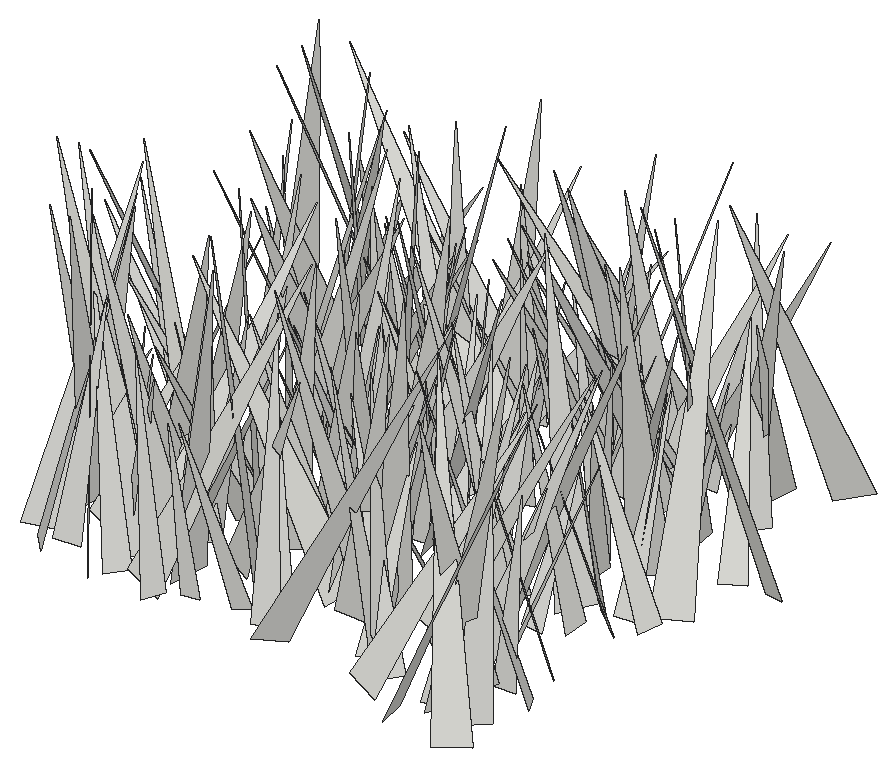
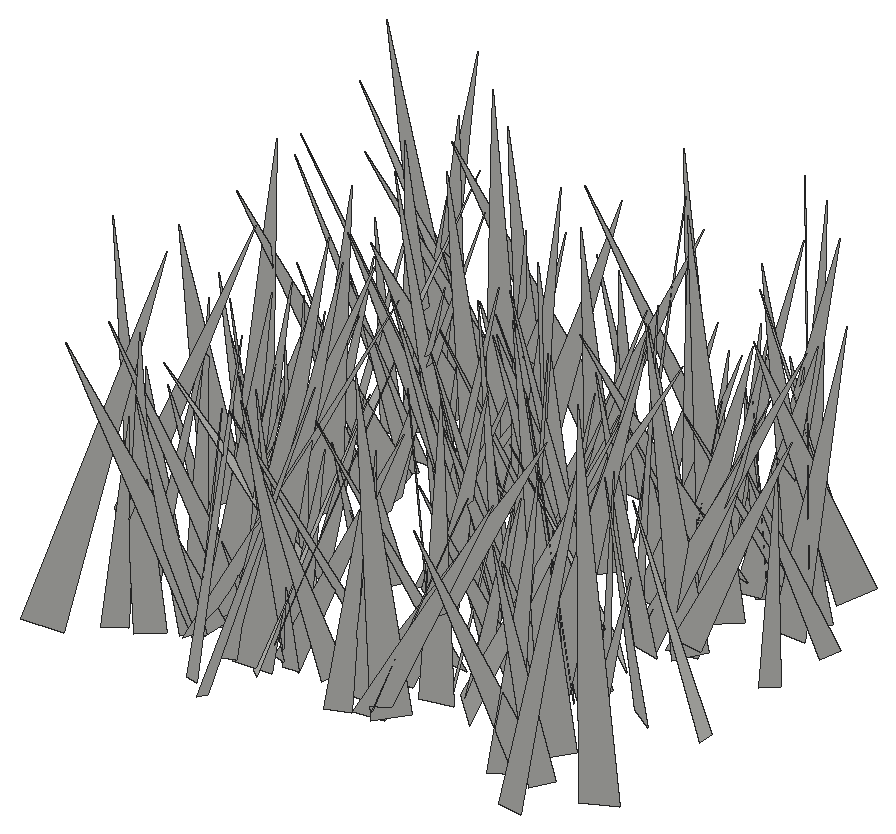
# SketchUp Ruby script. Lengths in inches.
U = 1.inch
M = Sketchup.active_model
def pt(a) = Geom::Point3d.new(a.map { |v| v * U })
def face(e, loops, mat)
  f = e.add_face(loops[0].map { |a| pt(a) })
  loops[1..].each { |l| e.add_face(l.map { |a| pt(a) }).erase! }
  f.material = f.back_material = mat if mat
  f
end
# faces: each face lists its corners as indices into pts; further lists are holes
def faces(e, pts, list, mat = nil) = list.each { |f| face(e, (f[0].is_a?(Array) ? f : [f]).map { |l| l.map { |i| pts[i] } }, mat) }
# xy, xz, yz: faces in a plane at the given z, y or x. An outline is a flat list of corners, or four numbers for a rectangle; further outlines are holes
def ring(l) = l.size == 4 ? [[l[0], l[1]], [l[2], l[1]], [l[2], l[3]], [l[0], l[3]]] : l.each_slice(2).to_a
def flat(e, list, mat, &to3) = list.each { |f| face(e, (f[0].is_a?(Array) ? f : [f]).map { |l| ring(l).map { |u, v| to3.(u, v) } }, mat) }
def xy(e, z, list, mat = nil) = flat(e, list, mat) { |x, y| [x, y, z] }
def xz(e, y, list, mat = nil) = flat(e, list, mat) { |x, z| [x, y, z] }
def yz(e, x, list, mat = nil) = flat(e, list, mat) { |y, z| [x, y, z] }
def lines(e, pts, list) = list.each { |a, b| e.add_line(pt(pts[a]), pt(pts[b])) }
# prism: a flat outline (further loops are holes) pulled along v
def prism(e, loops, v, mat = nil)
  f = face(e, loops, mat); d = Geom::Vector3d.new(v.map { |x| x * U })
  f.pushpull(f.normal.samedirection?(d) ? d.length : -d.length)
end
def box(e, o, s, mat = nil) = prism(e, [[o, [o[0] + s[0], o[1], o[2]], [o[0] + s[0], o[1] + s[1], o[2]], [o[0], o[1] + s[1], o[2]]]], [0, 0, s[2]], mat)
def at(x, y, z, deg = 0) = Geom::Transformation.translation(pt([x, y, z])) * Geom::Transformation.rotation(ORIGIN, Z_AXIS, deg.degrees)
def axes(o, x, y, z) = Geom::Transformation.new([*x, 0, *y, 0, *z, 0, *pt(o).to_a, 1])
def part(name) = M.definitions.add(name)
# library, detail: a bought-in or finely detailed component or shape, given as its bounding box
def library(name, o, s) = part(name).tap { |d| box(d.entities, o, s) }
def detail(e, o, s) = box(e.add_group.entities, o, s)
def put(e, d, t, mat = nil) = e.add_instance(d, t).tap { |i| i.material = mat if mat }
def group(e, t, mat = nil) = e.add_group.tap { |g| g.transformation = t; g.material = mat if mat }.entities
root = M.entities
c1 = part("fur_instance\#9")
p = [[0.8125,0,1.79],[0.67,-0.02,1.48],[0,-0.11,0],[0,0.11,0]]
faces(c1.entities,p,[[0,1,2,3]])
put(root,c1,axes([134.09,378.43,-27.1],[5.76412,-4.56343,1.38579],[-4.26746,-5.90574,-1.69745],[-2.12934,-0.51736,7.15322]))
put(root,c1,axes([135.99,374.47,-27.1],[-2.86004,7.00076,0.77945],[7.00763,2.7424,1.08181],[-0.71502,-1.12544,7.48466]))
put(root,c1,axes([132.64,375.04,-27.1],[7.12948,2.21776,0.41944],[2.17259,-7.11974,0.71624],[-0.61174,0.56098,7.43203]))
put(root,c1,axes([133.92,376.66,-27.1],[7.67247,-2.21843,2.0813],[-2.41925,-7.8734,0.52613],[-1.84403,1.09916,7.96941]))
put(root,c1,axes([116.74,376.78,-27.1],[-5.8561,-4.67693,3.47291],[-5.12361,6.47844,0.0849],[2.77191,2.09401,7.49403]))
put(root,c1,axes([120.1,376.48,-27.1],[-4.33048,1.8912,1.2808],[1.94847,4.49129,-0.04381],[1.19187,-0.47097,4.72523]))
put(root,c1,axes([123.3,377.78,-27.1],[0.25989,-4.12749,1.06746],[-4.12688,-0.51192,-0.97467],[-1.06982,0.97209,4.01917]))
put(root,c1,axes([121.22,377.3,-27.1],[0.17752,-3.57602,1.3313],[-3.7929,-0.31113,-0.32997],[-0.41733,1.30655,3.56518]))
put(root,c1,axes([120.11,378.6,-27.1],[7.47084,-2.00529,1.5784],[-1.88161,-7.62701,-0.78379],[-1.72397,-0.36551,7.69548]))
put(root,c1,axes([130.46,376,-27.1],[1.42855,6.69806,0.59183],[6.31436,-1.12829,-2.47201],[2.31152,-1.05735,6.38701]))
put(root,c1,axes([125.57,376.6,-27.1],[7.23014,-2.66142,0.8801],[-2.79977,-6.73645,2.62947],[0.1379,2.76941,7.24182]))
put(root,c1,axes([130.05,377.68,-27.1],[-5.84783,-0.54956,0.92386],[-0.66437,5.86496,-0.71656],[0.84507,0.80798,5.82972]))
put(root,c1,axes([135.58,376.33,-27.1],[-6.65914,2.85732,1.17721],[2.6023,6.69305,-1.52492],[1.66678,0.96593,7.084]))
put(root,c1,axes([115.02,377.66,-27.1],[-0.99114,4.85366,1.48422],[5.00835,1.18049,-0.51592],[0.82303,-1.33855,4.92689]))
put(root,c1,axes([119.22,376.96,-27.1],[1.74287,7.71217,1.36191],[7.45298,-1.20484,-2.71503],[2.4053,-1.85492,7.42588]))
put(root,c1,axes([119.18,379.17,-27.1],[-7.26017,0.65472,1.63239],[0.85,7.37598,0.82207],[1.53976,-0.9847,7.24313]))
put(root,c1,axes([113.81,381.06,-27.1],[7.57168,-2.77915,1.4038],[-2.39268,-7.55557,-2.05259],[-1.99233,-1.48808,7.80006]))
put(root,c1,axes([117.86,377.12,-27.1],[-5.44212,1.96061,0.21811],[1.90755,5.39324,-0.88463],[0.50284,0.7598,5.71648]))
put(root,c1,axes([130.01,377.82,-27.1],[-5.54219,0.95074,1.40051],[0.80502,5.69802,-0.68242],[1.48905,0.4581,5.58158]))
put(root,c1,axes([124.8125,377.26,-27.1],[-0.46142,6.00885,1.03301],[6.04976,0.32253,0.82618],[-0.75742,-1.08443,5.96964]))
put(root,c1,axes([136.26,378.83,-27.1],[-5.87124,-3.56524,0.53214],[-3.58838,5.68376,-1.51131],[-0.34307,1.5651,6.70063]))
put(root,c1,axes([130.94,377.24,-27.1],[-1.18961,5.30841,0.21099],[4.92708,1.02155,2.07828],[-1.98686,-0.64508,5.02744]))
put(root,c1,axes([127,379.875,-27.1],[2.07554,-6.96607,1.71735],[-7.11885,-1.77704,1.39545],[0.89291,2.02467,7.13349]))
put(root,c1,axes([122.99,379.21,-27.1],[-6.35073,-3.49942,2.22612],[-3.7296,6.59945,-0.26567],[1.81428,1.31702,7.24617]))
put(root,c1,axes([134.78,379.1,-27.1],[-0.53957,3.97433,2.02364],[4.38519,0.84425,-0.48882],[0.81275,-1.91664,3.98089]))
put(root,c1,axes([114.22,377.01,-27.1],[5.15399,5.0376,1.12923],[4.93282,-5.27609,1.02292],[-1.5231,-0.04087,7.13405]))
put(root,c1,axes([124.59,378.55,-27.1],[-2.6188,2.85202,1.01974],[2.95253,2.70449,0.01846],[0.67563,-0.76402,3.87193]))
put(root,c1,axes([129.3,377.81,-27.1],[-2.23012,3.65012,0.738],[3.54975,2.34365,-0.86487],[1.12574,-0.15918,4.18913]))
put(root,c1,axes([116.7,379.11,-27.1],[2.33806,3.32528,1.40975],[3.5899,-2.32407,-0.47188],[-0.3968,-1.43269,4.03749]))
put(root,c1,axes([121.08,380.21,-27.1],[-0.06945,-5.66946,1.63507],[-5.27402,0.7929,2.5253],[2.64594,1.43164,5.07647]))
put(root,c1,axes([116.05,380.35,-27.1],[-0.58442,-4.16845,1.10453],[-3.96593,0.95723,1.51414],[1.69333,0.80327,3.92746]))
put(root,c1,axes([127.69,380.28,-27.1],[-1.28539,6.13898,3.44989],[6.89976,0.39684,1.86462],[-1.40785,-3.66012,5.98853]))
put(root,c1,axes([127.63,381.2,-27.1],[3.37968,-7.43588,1.46776],[-7.57694,-3.27406,0.85991],[0.19143,1.6903,8.12251]))
put(root,c1,axes([125.64,380.97,-27.1],[-6.93796,2.79801,1.11968],[3.01121,6.55067,2.28891],[0.12298,-2.54512,7.12215]))
put(root,c1,axes([116.3,380.35,-27.1],[-4.3642,6.37446,3.0679],[7.06974,4.05938,1.62241],[0.25406,-3.46117,7.553]))
put(root,c1,axes([135.3,381.24,-27.1],[-3.21192,-3.98216,0.77509],[-3.98629,3.28152,0.34045],[0.75355,0.38579,5.10471]))
put(root,c1,axes([133.55,376.53,-27.1],[-6.0414,2.82747,0.77084],[2.14541,5.47009,-3.25002],[1.99649,2.67784,5.82499]))
put(root,c1,axes([115.99,380.21,-27.1],[3.13173,2.6382,1.54856],[2.8558,-3.31576,-0.12654],[-1.0966,-1.10068,4.0929]))
put(root,c1,axes([113.33,380.84,-27.1],[4.2743,-5.66959,1.70794],[-5.91958,-4.14155,1.06631],[-0.14077,2.00854,7.01974]))
put(root,c1,axes([117.75,382.05,-27.1],[3.73697,-5.4189,0.58942],[-5.45085,-3.71358,0.41766],[0.01126,0.72231,6.56925]))
put(root,c1,axes([116.83,382.71,-27.1],[4.42124,-3.27,0.9733],[-2.9097,-4.44582,-1.71927],[-1.78153,-0.85401,5.22344]))
put(root,c1,axes([117.72,378.53,-27.1],[-0.98442,7.82804,0.7856],[7.24103,0.59195,3.17514],[-3.07617,-1.11168,7.22258]))
put(root,c1,axes([130.6,380.02,-27.1],[4.59981,5.90875,0.46757],[5.722,-4.27232,-2.30133],[1.54616,-1.76752,7.12569]))
put(root,c1,axes([113.44,378.05,-27.1],[-5.30404,4.85737,1.41696],[4.30663,5.41145,-2.42976],[2.65607,0.92563,6.76928]))
put(root,c1,axes([113.57,381.97,-27.1],[0.65749,-6.30029,1.7132],[-6.47052,-0.85883,-0.67511],[-0.87239,1.62165,6.29842]))
put(root,c1,axes([124.79,380.67,-27.1],[2.82445,3.52777,0.66946],[3.53756,-2.58781,-1.2883],[0.61561,-1.31488,4.33162]))
put(root,c1,axes([116.1,382.74,-27.1],[3.30529,-7.09092,0.75642],[-7.06387,-3.14139,1.41833],[0.97724,1.27626,7.69379]))
put(root,c1,axes([119.27,383.22,-27.1],[0.9036,-5.03288,0.01557],[-4.93923,-0.88981,-0.97923],[-0.96652,-0.158,5.01871]))
put(root,c1,axes([124.92,381.69,-27.1],[-5.6933,-0.47947,0.5538],[-0.44449,5.71072,0.37467],[0.58224,-0.32872,5.70116]))
put(root,c1,axes([118.86,381.36,-27.1],[4.80209,-1.99507,1.20954],[-2.10711,-4.89697,0.2883],[-1.00169,0.73669,5.19204]))
put(root,c1,axes([132.38,381.06,-27.1],[0.51441,-3.71167,1.78135],[-3.92489,0.09986,1.3415],[1.24297,1.85145,3.49879]))
put(root,c1,axes([132.69,380.19,-27.1],[2.40606,6.39383,1.08481],[6.38564,-2.13376,-1.58675],[1.13207,-1.55339,6.64473]))
put(root,c1,axes([114.79,379.82,-27.1],[1.15422,4.7345,0.08294],[4.6056,-1.10261,-1.15208],[1.10037,-0.35121,4.73502]))
put(root,c1,axes([118.68,380.27,-27.1],[4.79219,0.94532,0.41054],[0.81575,-4.67249,1.23678],[-0.62985,1.14081,4.72537]))
put(root,c1,axes([128.04,380.29,-27.1],[5.65388,1.0827,1.74004],[0.6959,-5.81697,1.3583],[-1.92762,1.07564,5.59407]))
put(root,c1,axes([121.86,382.43,-27.1],[5.17414,-4.36417,1.70527],[-4.54977,-5.28673,0.27499],[-1.1196,1.31532,6.76329]))
put(root,c1,axes([127.16,380.84,-27.1],[-1.66344,3.87519,0.54462],[3.91265,1.65754,0.1564],[0.06977,-0.56232,4.21422]))
put(root,c1,axes([129.25,382.64,-27.1],[-2.36065,-3.34559,0.0438],[-3.13879,2.19578,-1.44709],[-1.15883,0.86782,3.83035]))
put(root,c1,axes([111.43,382.11,-27.1],[2.74116,-2.85153,0.16279],[-2.64199,-2.44575,1.64616],[1.08517,1.2485,3.59657]))
put(root,c1,axes([117.92,383.03,-27.1],[-3.40624,-2.616,1.08161],[-2.59295,3.56228,0.44999],[1.13575,0.28715,4.27123]))
put(root,c1,axes([129.46,381.14,-27.1],[0.97735,4.73028,0.44464],[4.65378,-0.86171,-1.06216],[0.95682,-0.64061,4.71196]))
put(root,c1,axes([132.86,382.27,-27.1],[4.03846,2.29721,0.25382],[2.30928,-3.98992,-0.63131],[0.09403,-0.6739,4.60302]))
put(root,c1,axes([119.08,380.96,-27.1],[-0.71343,7.62578,1.29035],[7.14993,0.15622,3.02994],[-2.94889,-1.46615,7.03427]))
put(root,c1,axes([118.04,384.85,-27.1],[-5.4355,-1.48683,0.1699],[-1.41481,5.31415,1.24191],[0.48767,-1.15472,5.49664]))
put(root,c1,axes([129.49,382.84,-27.1],[-4.34694,-0.07841,1.0456],[-0.20123,4.43859,-0.5037],[1.02905,0.53671,4.31837]))
put(root,c1,axes([124.08,384.87,-27.1],[-1.04012,-7.65192,1.88155],[-7.84849,1.17518,0.4406],[0.70237,1.80029,7.70971]))
put(root,c1,axes([117.26,380.5,-27.1],[-0.93463,7.10607,0.24964],[6.82555,0.96718,-1.97702],[1.99262,0.02006,6.88921]))
put(root,c1,axes([123.86,384,-27.1],[-2.53875,-3.10556,0.31926],[-3.0835,2.42999,-0.88252],[-0.48832,0.80145,3.91291]))
put(root,c1,axes([121.82,384.92,-27.1],[2.30675,-6.01681,0.97122],[-6.03702,-2.11321,1.24701],[0.83643,1.34116,6.32203]))
put(root,c1,axes([125.18,382.68,-27.1],[4.28943,0.41298,0.87796],[0.18379,-4.25331,1.1028],[-0.95267,1.03894,4.16576]))
put(root,c1,axes([133.97,384.39,-27.1],[-5.16901,0.01394,1.37798],[0.15537,5.32107,0.52899],[1.36927,-0.55116,5.14189]))
put(root,c1,axes([117.46,382.4375,-27.1],[-6.47288,0.26814,0.01301],[0.25719,6.28405,-1.55397],[0.07694,1.55212,6.2893]))
put(root,c1,axes([131.41,383.42,-27.1],[-5.82181,0.2065,0.70872],[0.14567,5.84473,-0.50632],[0.72368,0.48471,5.80343]))
put(root,c1,axes([123.96,382.45,-27.1],[4.21835,1.12148,1.8478],[0.48542,-4.44001,1.58659],[-2.10629,1.22277,4.06632]))
put(root,c1,axes([111.69,385.42,-27.1],[3.7269,-2.05729,0.24824],[-1.97365,-3.67974,-0.86491],[-0.63149,-0.64103,4.16823]))
put(root,c1,axes([131.12,384.55,-27.1],[-7.49054,-0.65717,0.9559],[-0.61994,7.54719,0.33069],[0.98046,-0.24861,7.51203]))
put(root,c1,axes([118.9375,384.23,-27.1],[-4.32305,-4.69404,2.5219],[-5.10648,4.57733,-0.23372],[1.52244,2.02405,6.37716]))
put(root,c1,axes([117.51,385.6,-27.1],[-3.5976,-6.50533,0.64098],[-6.34012,3.29439,-2.15004],[-1.59153,1.58132,7.11613]))
put(root,c1,axes([126.53,385.39,-27.1],[2.79226,2.81825,2.22878],[3.51982,-2.71249,-0.9798],[-0.72174,-2.32521,3.84438]))
put(root,c1,axes([125.8,386.2,-27.1],[7.87771,-0.03675,0.30438],[0.03502,-7.66773,-1.83222],[-0.30459,-1.83219,7.66177]))
put(root,c1,axes([135.26,384.93,-27.1],[-2.96371,-3.18096,0.56073],[-3.21747,2.84043,-0.89238],[-0.28422,1.01488,4.25508]))
put(root,c1,axes([123.08,383.51,-27.1],[2.64419,5.03318,0.33977],[4.95036,-2.51506,-1.26831],[0.97076,-0.88412,5.54221]))
put(root,c1,axes([115.47,385.45,-27.1],[5.59181,-3.37862,1.09906],[-3.46581,-5.63815,0.30113],[-0.78177,0.82912,6.52631]))
put(root,c1,axes([132.68,383.39,-27.1],[-0.04754,4.40868,0.34675],[4.41199,0.07095,-0.29716],[0.30179,-0.34273,4.39891]))
put(root,c1,axes([124.6,385.89,-27.1],[3.42079,-7.2545,1.9343],[-7.49487,-3.17419,1.34998],[0.44283,2.31686,7.90614]))
put(root,c1,axes([131.85,382.36,-27.1],[7.63616,1.08232,1.22596],[0.61242,-7.3209,2.64853],[-1.51635,2.49367,7.24345]))
put(root,c1,axes([115.83,385.51,-27.1],[-4.20776,3.77593,1.0344],[3.85861,3.7428,2.0336],[-0.66241,-2.18328,5.27517]))
put(root,c1,axes([124.6875,385.53,-27.1],[2.97768,-2.23657,0.59018],[-2.29034,-2.98547,0.24174],[-0.32391,0.5494,3.71623]))
put(root,c1,axes([122.9,383.22,-27.1],[-3.04551,1.64304,1.0176],[0.80196,2.80235,-2.12461],[1.7584,1.56764,2.73144]))
put(root,c1,axes([134.17,385.82,-27.1],[-2.56443,-3.19615,1.19823],[-3.34404,2.653,-0.08027],[0.6845,0.98675,4.09698]))
put(root,c1,axes([124.12,382.03,-27.1],[-7.01528,2.7432,0.95764],[2.14491,6.5776,-3.12905],[1.96,2.6204,6.85188]))
put(root,c1,axes([122.43,386.53,-27.1],[-0.63614,-4.28295,0.71253],[-4.25699,0.4736,-0.95381],[-0.85404,0.8295,4.22357]))
put(root,c1,axes([133.02,385.6,-27.1],[-6.40886,3.74132,2.19702],[3.96061,6.64492,0.23769],[1.77143,-1.32114,7.41717]))
put(root,c1,axes([136.16,386.09,-27.1],[-4.59292,1.38597,0.57425],[1.45174,4.5724,0.57548],[0.37836,-0.71958,4.76284]))
put(root,c1,axes([128.11,384.11,-27.1],[-0.8094,5.47668,0.09308],[5.43232,0.79056,0.72297],[-0.70181,-0.19701,5.48875]))
put(root,c1,axes([122.48,386.94,-27.1],[-4.6508,-5.63712,0.37429],[-5.36466,4.25457,-2.58191],[-1.77136,1.91537,6.83673]))
put(root,c1,axes([122.11,386.6875,-27.1],[-1.05055,-3.99645,1.56356],[-4.12582,0.49771,-1.49997],[-1.18067,1.81677,3.85037]))
put(root,c1,axes([123.86,386.32,-27.1],[0.25719,7.17904,2.90731],[6.91163,1.10018,-3.3281],[3.49578,-2.70337,6.36621]))
put(root,c1,axes([126.64,387.42,-27.1],[-5.33847,-0.05884,0.40473],[-0.0096,5.31499,0.64603],[0.40887,-0.64342,5.29956]))
put(root,c1,axes([132.07,388.16,-27.1],[4.60045,-1.39498,0.802],[-1.20201,-4.59424,-1.0961],[-1.06973,-0.83684,4.68067]))
put(root,c1,axes([116.97,386.22,-27.1],[1.78136,5.8506,1.71123],[6.09225,-1.76893,-0.29408],[-0.20572,-1.72409,6.10871]))
put(root,c1,axes([125.85,388.08,-27.1],[-3.47477,-5.64058,1.59223],[-5.83486,3.50381,-0.32112],[0.55295,1.52727,6.61718]))
put(root,c1,axes([135,386.13,-27.1],[-1.136,4.49998,0.83575],[4.53043,1.22799,-0.4539],[0.65076,-0.69355,4.61891]))
put(root,c1,axes([133.57,389.33,-27.1],[4.47344,-6.57845,1.38646],[-6.62258,-4.59864,-0.45163],[-1.15746,0.88686,7.94253]))
put(root,c1,axes([134.4,387.4,-27.1],[4.12014,1.91723,1.34742],[2.03951,-4.27599,-0.15214],[-1.154,-0.71202,4.54182]))
put(root,c1,axes([117.89,387.68,-27.1],[2.9133,6.77269,2.26525],[7.08174,-2.424,-1.8604],[0.9217,-2.7826,7.13411]))
put(root,c1,axes([117.75,390.95,-27.1],[5.40513,-4.44008,1.03103],[-3.91993,-5.34397,-2.46351],[-2.32626,-1.31164,6.54682]))
put(root,c1,axes([123.17,387.11,-27.1],[-6.34859,-2.07949,3.15929],[-2.7531,6.77324,-1.07409],[2.59343,2.09974,6.59357]))
put(root,c1,axes([122.86,386.875,-27.1],[5.61181,2.09612,1.30854],[1.89864,-5.73587,1.04566],[-1.58152,0.55181,5.89854]))
put(root,c1,axes([124.49,386.4375,-27.1],[2.31766,5.02687,0.82298],[4.84651,-2.45447,1.34356],[-1.56781,-0.15629,5.3699]))
put(root,c1,axes([122.39,387.22,-27.1],[-5.96382,1.04535,0.88629],[0.82737,5.90096,-1.39268],[1.09259,1.23747,5.8924]))
put(root,c1,axes([127.43,388.02,-27.1],[-2.50227,2.59124,1.1484],[2.47228,2.74461,-0.80603],[1.38608,-0.21748,3.51087]))
put(root,c1,axes([116.39,389.98,-27.1],[2.55754,-6.5759,0.86107],[-6.14173,-2.00015,2.96707],[2.50263,1.81158,6.40156]))
put(root,c1,axes([131.16,389.52,-27.1],[-1.15878,-4.12917,1.68532],[-4.31214,1.48176,0.66553],[1.13832,1.40977,4.23673]))
put(root,c1,axes([130.01,389.49,-27.1],[-1.05409,-4.02831,1.60299],[-4.27873,0.70037,-1.05356],[-0.69957,1.78611,4.02845]))
put(root,c1,axes([136.31,387.1875,-27.1],[-5.32969,5.59283,1.04722],[5.46672,5.43108,-1.18331],[1.57839,0.07463,7.63447]))
put(root,c1,axes([111.1,389.97,-27.1],[4.64757,1.11707,0.03174],[1.0994,-4.54603,-0.98676],[0.20042,-0.96672,4.67697]))
put(root,c1,axes([124.5,389.7,-27.1],[3.53151,3.08583,1.68165],[3.37882,-3.63698,-0.42174],[-0.96639,-1.43941,4.67077]))
put(root,c1,axes([117.125,388.43,-27.1],[2.66286,4.62658,1.9724],[4.32664,-3.24515,1.77077],[-2.56433,-0.67099,5.03592]))
put(root,c1,axes([119.32,390.47,-27.1],[3.99412,4.65299,3.2629],[5.30006,-4.48907,-0.08624],[-2.05092,-2.53923,6.13155]))
put(root,c1,axes([116.52,393.14,-27.1],[4.04445,-6.42376,0.8146],[-6.13253,-4.10829,-1.94934],[-2.07854,-0.37835,7.33638]))
put(root,c1,axes([122.39,388.78,-27.1],[7.1658,2.76652,1.69463],[2.58302,-7.35112,1.0785],[-1.96302,0.42601,7.60521]))
put(root,c1,axes([117.43,387.03,-27.1],[4.44404,5.53922,0.27989],[5.13876,-4.2472,2.46279],[-2.08674,1.3376,6.66087]))
put(root,c1,axes([120.92,391.12,-27.1],[1.65267,-3.08975,1.39314],[-3.11179,-1.99748,-0.7386],[-1.34319,0.82596,3.42525]))
put(root,c1,axes([130.18,392.33,-27.1],[6.41369,-0.07562,0.05633],[-0.05586,-6.13403,-1.87481],[-0.07597,-1.87412,6.13403]))
put(root,c1,axes([133.49,392.46,-27.1],[5.23051,-1.10724,0.78196],[-0.81536,-5.06,-1.7109],[-1.08287,-1.53819,5.06527]))
put(root,c1,axes([138.26,390.87,-27.1],[-4.4516,-6.59475,1.62319],[-6.65602,3.85048,-2.61027],[-1.35017,2.76139,7.51625]))
put(root,c1,axes([133.38,389.74,-27.1],[-5.0928,-0.09663,0.30052],[-0.16718,4.94609,-1.24277],[0.26777,1.25023,4.93978]))
put(root,c1,axes([117.98,391.06,-27.1],[4.10331,-3.61689,0.17449],[-3.47529,-3.85943,1.7253],[1.0172,1.40442,5.19061]))
put(root,c1,axes([124.27,389.5,-27.1],[-6.63605,2.7216,0.19643],[2.70208,6.62626,-0.52374],[0.38006,0.41041,7.15332]))
put(root,c1,axes([134.29,390.28,-27.1],[3.78689,-0.0231,1.24793],[-0.32688,-3.86581,0.92039],[-1.20458,0.97644,3.67342]))
put(root,c1,axes([130.89,394.11,-27.1],[0.06912,-7.57158,0.2529],[-7.42195,-0.11839,-1.51598],[-1.51902,0.23392,7.41859]))
put(root,c1,axes([113.92,390.32,-27.1],[2.58353,5.00263,1.49189],[5.09313,-2.78069,0.50442],[-1.14546,-1.08079,5.60772]))
put(root,c1,axes([130.99,393.18,-27.1],[5.55902,-2.83125,1.90418],[-2.404,-5.83322,-1.65498],[-2.42129,-0.70867,6.01496]))
put(root,c1,axes([117.3,390.2,-27.1],[4.85297,5.01471,2.08252],[4.89411,-5.24941,1.23566],[-2.35199,-0.5761,6.86817]))
put(root,c1,axes([126.67,390.625,-27.1],[1.26657,4.59176,1.22685],[4.36989,-1.62436,1.56816],[-1.86909,-0.68616,4.4977]))
put(root,c1,axes([116.08,392.62,-27.1],[0.58274,-3.68979,0.92218],[-3.78198,-0.46356,0.53511],[0.40205,0.98748,3.697]))
put(root,c1,axes([124.22,392.13,-27.1],[2.61371,2.45973,0.53308],[2.49517,-2.43181,-1.01309],[0.32949,-1.09634,3.44317]))
put(root,c1,axes([134.39,394.05,-27.1],[-1.58112,-4.73276,0.31075],[-4.65779,1.61119,0.83937],[0.89473,0.02406,4.91878]))
put(root,c1,axes([120.67,393.18,-27.1],[-3.88391,-3.01754,1.00768],[-2.99103,4.00531,0.46572],[1.08383,0.24005,4.89626]))
put(root,c1,axes([114.58,394.39,-27.1],[8.18505,-1.50624,0.16494],[-1.43272,-7.98824,-1.85106],[-0.49323,-1.79175,8.11402]))
put(root,c1,axes([125.53,391.625,-27.1],[4.20313,-0.16718,1.34956],[-0.39887,-4.34286,0.70427],[-1.30006,0.79192,4.14708]))
put(root,c1,axes([136.42,390.7,-27.1],[-3.1637,4.01487,0.30871],[3.99884,3.17867,-0.35895],[0.47305,-0.01931,5.09895]))
put(root,c1,axes([128.39,393.97,-27.1],[-5.1626,-2.88411,0.4563],[-2.82641,5.16852,0.6903],[0.7333,-0.3834,5.87316]))
put(root,c1,axes([130.2,394.53,-27.1],[2.51881,-4.55482,0.15905],[-4.51842,-2.51942,-0.59372],[-0.59628,-0.14918,5.17091]))
put(root,c1,axes([118.09,391.78,-27.1],[4.70172,-1.10111,0.26171],[-1.12934,-4.49092,1.39405],[0.07438,1.41645,4.62334]))
put(root,c1,axes([114.15,393.07,-27.1],[-0.09942,-3.58739,1.13729],[-3.70553,-0.10534,-0.65623],[-0.65715,1.13676,3.52826]))
put(root,c1,axes([131.42,394.98,-27.1],[-3.70308,-3.24105,0.05421],[-3.08159,3.54543,1.46762],[1.00557,-1.07036,4.69716]))
put(root,c1,axes([128.72,392.23,-27.1],[-0.54656,4.2534,1.19948],[4.32093,0.26075,1.04426],[-0.92722,-1.29209,4.15928]))
put(root,c1,axes([130.02,393.08,-27.1],[-3.10303,1.40825,1.48641],[1.65077,3.31728,0.3033],[1.21143,-0.91317,3.39411]))
put(root,c1,axes([119.58,393.15,-27.1],[-3.58724,1.8714,1.40372],[2.1412,3.66165,0.59026],[0.94225,-1.19623,4.00275]))
put(root,c1,axes([128.3,396.13,-27.1],[6.29678,-5.28708,1.00032],[-4.88133,-6.26054,-2.36253],[-2.26416,-1.20654,7.87535]))
put(root,c1,axes([119.46,393.89,-27.1],[-4.9129,-5.75828,0.52895],[-5.68371,4.68095,-1.83254],[-1.06438,1.58274,7.34412]))
put(root,c1,axes([131,395.65,-27.1],[-8.10416,-1.22815,0.06312],[-1.16757,7.81624,2.17553],[0.38615,-2.14192,7.90272]))
put(root,c1,axes([127.72,396.29,-27.1],[0.59961,-8.00132,0.48644],[-8.01433,-0.60861,-0.13198],[-0.1682,0.47514,8.02267]))
put(root,c1,axes([126.86,395.32,-27.1],[0.11807,-5.18176,0.38422],[-4.95689,-0.22756,-1.54584],[-1.55804,0.33133,4.94722]))
put(root,c1,axes([117.26,392.69,-27.1],[-0.85461,3.70026,0.75554],[3.7566,0.91253,-0.21994],[0.38824,-0.68446,3.79129]))
put(root,c1,axes([130.57,394.62,-27.1],[4.49335,-4.83843,2.48866],[-4.8443,-5.0271,-1.02712],[-2.47721,1.05444,6.5227]))
put(root,c1,axes([121.8,391.55,-27.1],[1.69788,6.23349,0.03172],[6.16311,-1.67374,-0.97718],[0.93461,-0.28707,6.38626]))
put(root,c1,axes([128.71,393.38,-27.1],[0.78552,4.64999,1.51438],[4.88897,-0.70993,-0.35606],[0.11721,-1.55126,4.70241]))
put(root,c1,axes([127.33,396.62,-27.1],[-4.17954,-4.03403,0.06779],[-3.83281,4.00041,1.74723],[1.26,-1.21235,5.53978]))
put(root,c1,axes([129.81,389.9,-27.1],[5.70548,5.18554,0.14342],[4.71826,-5.27598,3.06024],[-2.15603,2.1765,7.07653]))
put(root,c1,axes([120.68,394.11,-27.1],[-1.61639,5.70202,2.80279],[6.31476,1.76115,0.05886],[0.70173,-2.71416,5.92641]))
put(root,c1,axes([122.23,395.88,-27.1],[-4.07436,-2.22938,0.28557],[-2.14023,4.02883,0.91657],[0.68639,-0.67121,4.55307]))
put(root,c1,axes([132.32,396.65,-27.1],[0.1957,-7.90399,1.09327],[-7.43409,0.21668,2.89722],[2.89871,1.0893,7.35646]))
put(root,c1,axes([123.125,393.8,-27.1],[-5.23637,6.32875,0.17784],[5.87309,4.76933,3.20385],[-2.36465,-2.16904,7.5636]))
put(root,c1,axes([123.1875,393.6,-27.1],[2.725,5.40327,0.30402],[4.86473,-2.29653,-2.78814],[2.3711,-1.498,5.37096]))
put(root,c1,axes([126.53,395.5,-27.1],[-1.2496,-4.95098,2.04852],[-4.91628,1.89585,1.58307],[2.13046,1.47094,4.85465]))
put(root,c1,axes([115.35,396.8,-27.1],[4.3108,-3.69492,0.61953],[-3.55093,-4.33068,-1.12044],[-1.19463,-0.46051,5.56597]))
put(root,c1,axes([129.79,393.86,-27.1],[0.86928,6.52033,1.58307],[6.24969,-0.2059,-2.58369],[2.44176,-1.79425,6.04937]))
put(root,c1,axes([133.65,397.12,-27.1],[4.86782,-2.47433,0.4659],[-2.27673,-4.75873,-1.48527],[-1.07512,-1.1257,5.25471]))
put(root,c1,axes([111.08,396.39,-27.1],[1.84601,-7.44066,1.73932],[-7.59322,-1.58595,1.27441],[0.85535,1.97933,7.55956]))
put(root,c1,axes([123.16,396.88,-27.1],[2.62732,-3.98087,0.28129],[-3.95197,-2.64215,-0.47983],[-0.55532,-0.03119,4.74551]))
put(root,c1,axes([134.47,394.45,-27.1],[-5.32179,3.05618,1.70346],[3.04909,5.5718,-0.47069],[1.71611,-0.42222,6.11884]))
put(root,c1,axes([113.47,398.73,-27.1],[-3.16063,-7.46069,0.64697],[-7.21635,3.22195,1.90087],[2.00118,-0.16476,7.87643]))
put(root,c1,axes([122.98,395.68,-27.1],[-0.34045,4.62028,2.07312],[5.05885,0.21591,0.34957],[-0.23002,-2.08976,4.6196]))
put(root,c1,axes([124.91,394.9375,-27.1],[3.82826,-1.89723,1.31218],[-2.241,-3.66166,1.2438],[-0.54703,1.72325,4.08754]))
put(root,c1,axes([113.6875,396.54,-27.1],[3.31192,-3.28223,0.0309],[-3.2384,-3.26025,0.79144],[0.53549,0.5836,4.59516]))
put(root,c1,axes([121.27,396.05,-27.1],[5.02607,-4.57327,2.19343],[-4.92834,-5.13329,0.59007],[-1.19892,1.92923,6.76964]))
put(root,c1,axes([130.97,395.78,-27.1],[1.98838,-4.24744,1.75797],[-4.57109,-1.62434,1.24561],[0.4862,2.09896,4.52138]))
put(root,c1,axes([128.9,398.46,-27.1],[-3.46675,-5.54657,1.13696],[-5.08588,3.63649,2.23277],[2.48816,-0.29493,6.14797]))
put(root,c1,axes([130.86,395.61,-27.1],[-4.62696,-2.40171,1.71965],[-2.7299,4.69747,-0.78458],[1.12828,1.51649,5.15378]))
put(root,c1,axes([121.99,396.49,-27.1],[-4.61226,3.61546,0.79034],[3.61757,4.1381,2.18138],[-0.78062,-2.18488,5.43931]))
put(root,c1,axes([126.95,394.44,-27.1],[-5.68198,1.58826,2.45655],[1.00817,6.10119,-1.61279],[2.74605,1.04639,5.67506]))
put(root,c1,axes([135.83,398.73,-27.1],[3.52912,-6.81057,1.30534],[-6.45742,-3.76145,-2.16695],[-2.52774,0.10047,7.35818]))
put(root,c1,axes([127.82,399.17,-27.1],[-5.63617,-2.55407,1.20627],[-1.85262,5.37498,2.72438],[2.13217,-2.08115,5.55585]))
put(root,c1,axes([130.61,395.21,-27.1],[6.21247,-1.9108,0.54363],[-1.98453,-5.88708,1.9863],[0.09123,2.05733,6.18874]))
put(root,c1,axes([114.43,396.26,-27.1],[3.95823,-3.37287,0.12226],[-3.1364,-3.60629,2.0534],[1.24667,1.63622,4.7778]))
